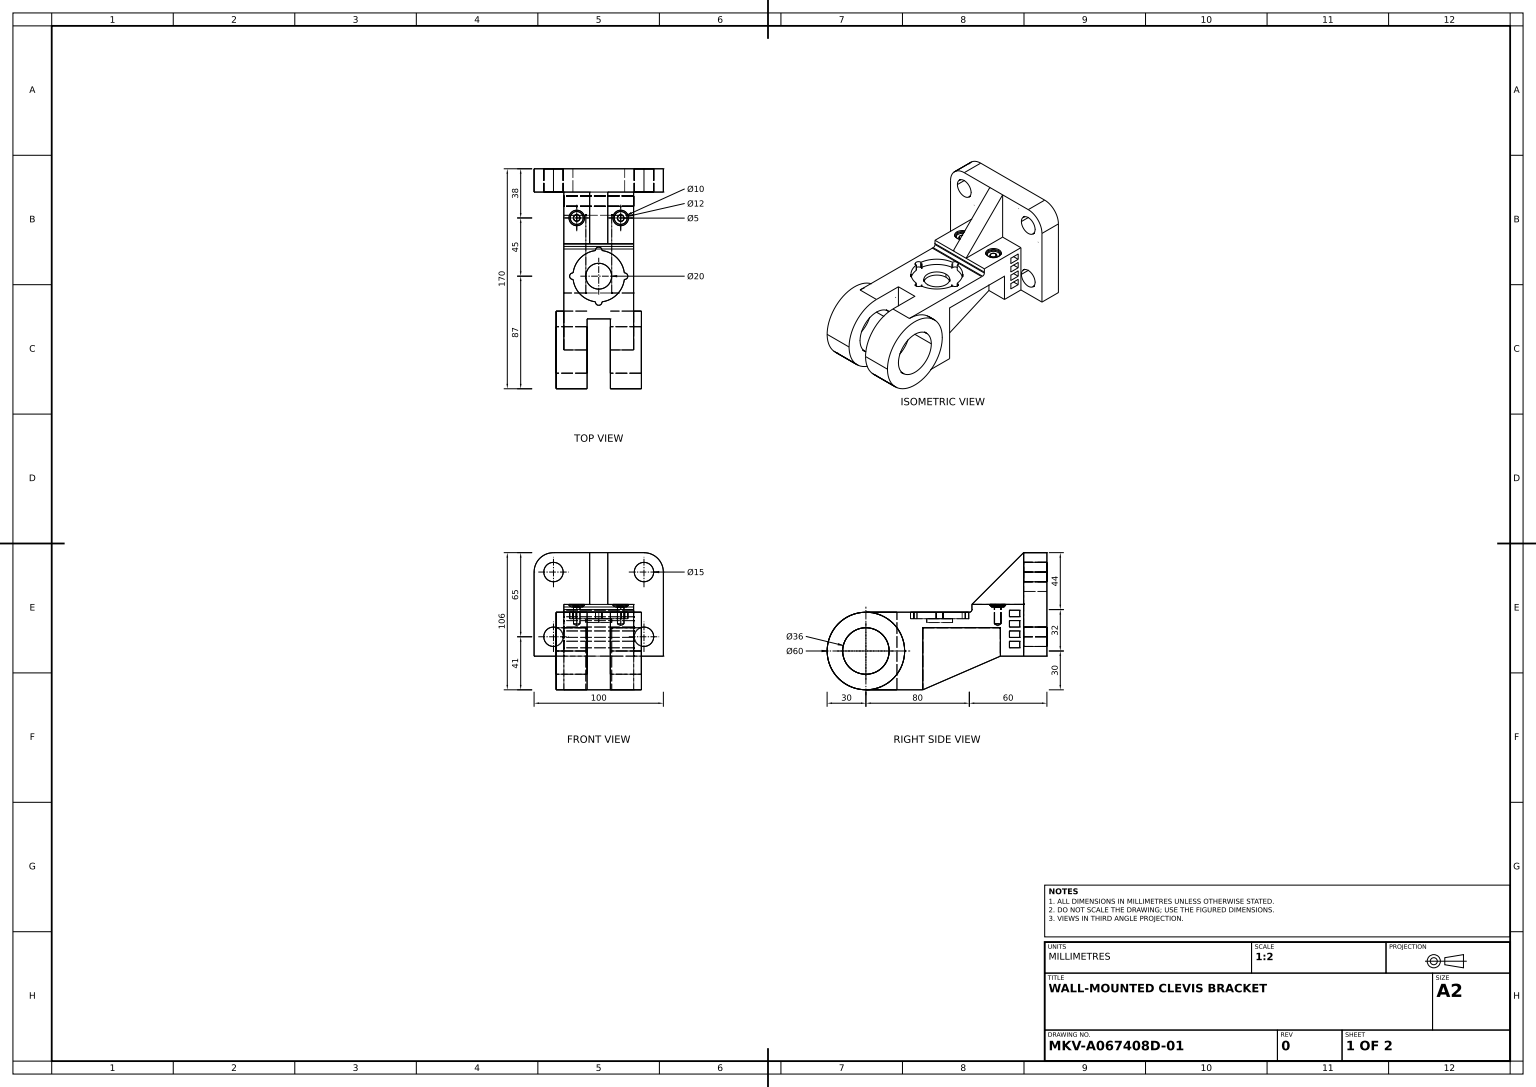
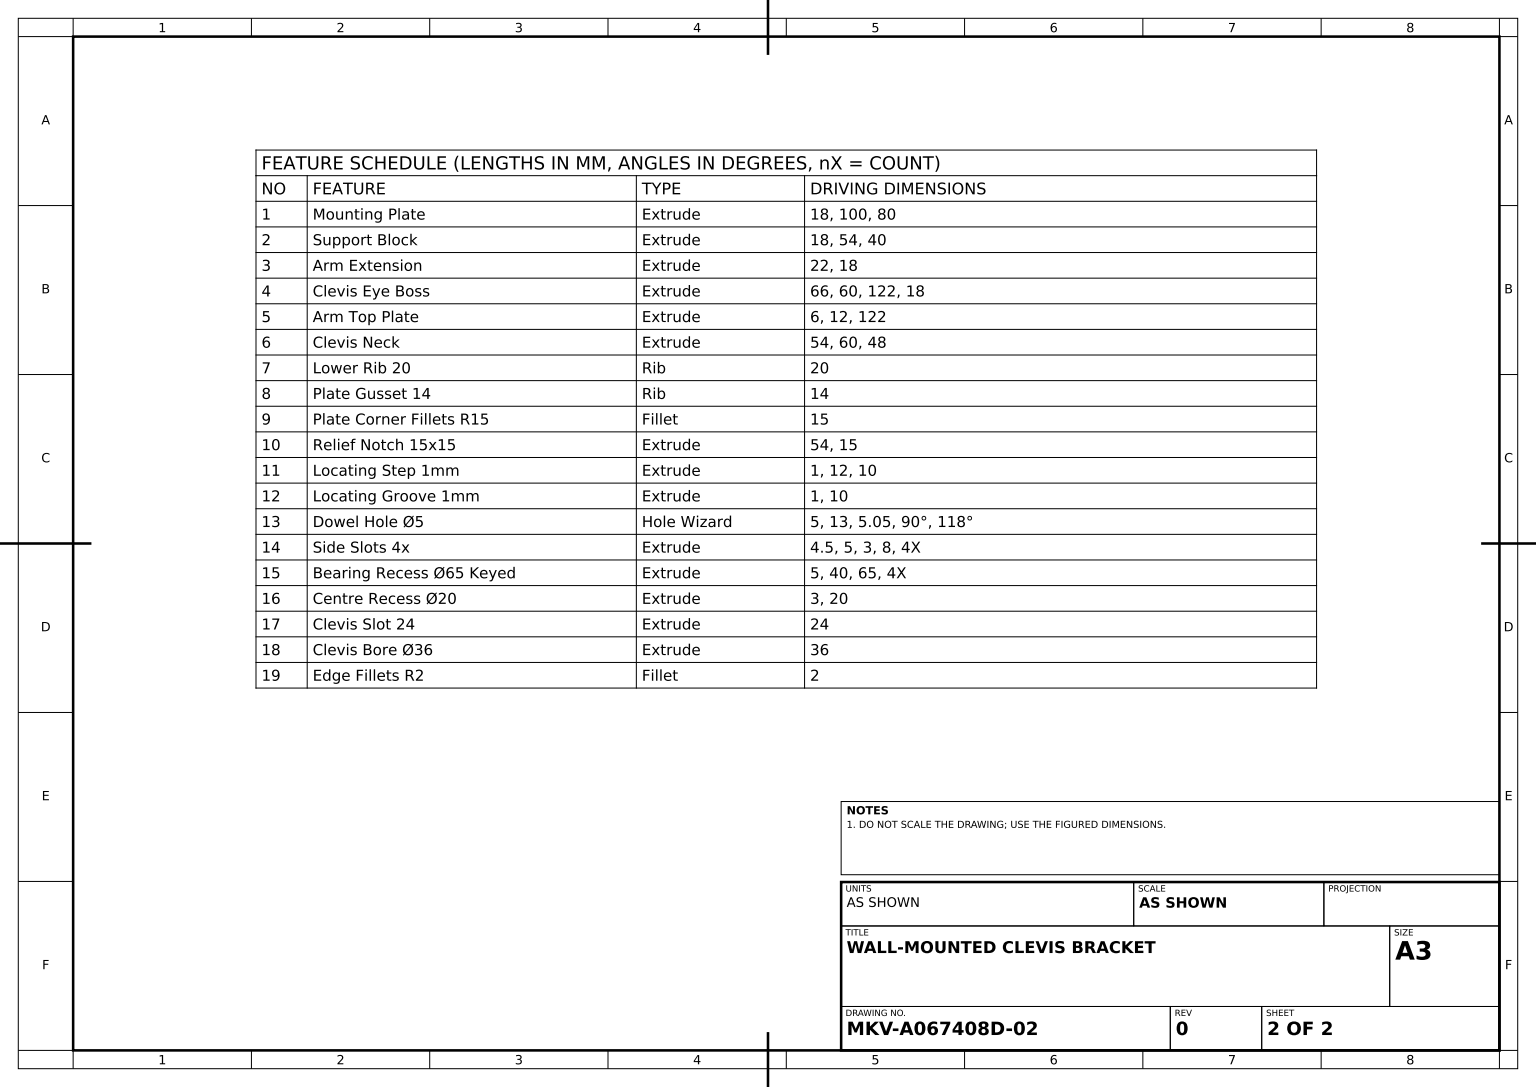
solid
v1 (-35,40,18)
v2 (-50,25,18)
e1 v1 v2 CIRCLE(AX(P(-35,25,18),D(0,0,1),D(-1,0,0)),15)
v3 (-35,40,0)
e2 v3 v1 LINE
v4 (-50,25,0)
e3 v4 v3 CIRCLE(AX(P(-35,25,0),D(0,0,-1),D(-1,0,0)),15)
e4 v2 v4 LINE
face CYL(AX(P(-35,25,18),D(0,0,-1),D(-1,0,0)),15) [-e1 -e2 -e3 -e4]
v5 (27,-12.5,29)
v6 (-27,-12.5,29)
e5 v5 v6 LINE
v7 (-27,-12.5,21)
e6 v6 v7 LINE
v8 (27,-12.5,21)
e7 v8 v7 LINE
e8 v5 v8 LINE
face PLANE(AX(P(50,-12.5,21),D(0,1,0),D(0,0,1))) rev [e5 e6 -e7 -e8]
v9 (20,-11,85.5)
v10 (20,-11,80.5)
e9 v9 v10 CIRCLE(AX(P(20,-11,83),D(0,1,0),D(0,0,1)),2.5)
v11 (20,-6,85.5)
e10 v9 v11 LINE
v12 (20,-6,80.5)
e11 v11 v12 CIRCLE(AX(P(20,-6,83),D(0,1,0),D(0,0,1)),2.5)
e12 v10 v12 LINE
face CYL(AX(P(20,-11,83),D(0,1,0),D(0,0,1)),2.5) rev [-e9 e10 e11 -e12]
v13 (27,-25.5,21)
v14 (27,-25.5,29)
e13 v13 v14 LINE
v15 (-27,-25.5,21)
e14 v13 v15 LINE
v16 (-27,-25.5,29)
e15 v15 v16 LINE
e16 v14 v16 LINE
face PLANE(AX(P(50,-25.5,21),D(0,-1,0),D(0,0,-1))) rev [-e13 e14 e15 -e16]
v17 (33,-36,122)
v18 (9,-36,122)
e17 v17 v18 LINE
v19 (9,-36,158)
e18 v19 v18 CIRCLE(AX(P(9,-36,140),D(1,0,0),D(0,0,-1)),18)
v20 (33,-36,158)
e19 v20 v19 LINE
e20 v20 v17 CIRCLE(AX(P(33,-36,140),D(1,0,0),D(0,0,-1)),18)
face CYL(AX(P(50,-36,140),D(-1,0,0),D(0,0,1)),18) rev [e17 -e18 -e19 e20]
v21 (27,-20.5,29)
v22 (-27,-20.5,29)
e21 v21 v22 LINE
e22 v14 v21 LINE
e23 v16 v22 LINE
face PLANE(AX(P(50,-20.5,29),D(0,0,1),D(1,0,0))) rev [-e21 -e22 e16 e23]
v23 (-17,-2,35.475)
v24 (-17,-2,40.525)
e24 v23 v24 CIRCLE(AX(P(-17,-2,38),D(0,1,0),D(0,0,1)),2.525)
v25 (-17,-2.025,40.5)
e25 v25 v24 LINE
v26 (-17,-2.025,35.5)
e26 v26 v25 CIRCLE(AX(P(-17,-2.025,38),D(0,1,0),D(0,0,1)),2.5)
e27 v26 v23 LINE
face CONE(AX(P(-17,-2,38),D(0,1,0),D(0,0,1)),2.525,0.785398163) rev [e24 -e25 -e26 e27]
v27 (12,-2,38)
v28 (12,-1,38)
e28 v27 v28 LINE
v29 (22,-2,38)
e29 v29 v27 CIRCLE(AX(P(17,-2,38),D(0,1,0),D(-1,0,0)),5)
v30 (22,-1,38)
e30 v29 v30 LINE
e31 v30 v28 CIRCLE(AX(P(17,-1,38),D(0,1,0),D(-1,0,0)),5)
face CYL(AX(P(17,-2,38),D(0,1,0),D(-1,0,0)),5) rev [-e28 -e29 e30 e31]
v31 (19.84375,-6,80.504888)
e32 v12 v31 CIRCLE(AX(P(20,-6,83),D(0,1,0),D(0,0,1)),2.5)
v32 (19.84375,-11,80.504888)
e33 v32 v31 LINE
e34 v10 v32 CIRCLE(AX(P(20,-11,83),D(0,1,0),D(0,0,1)),2.5)
face CYL(AX(P(20,-11,83),D(0,1,0),D(0,0,1)),2.5) rev [e32 -e33 -e34 e12]
v33 (17,-16.502152,38.121872)
v34 (17,-15,40.621872)
e35 v33 v34 LINE
v35 (17,-15,35.621872)
e36 v33 v35 LINE
e37 v35 v34 CIRCLE(AX(P(17,-15,38.121872),D(0,1,0),D(0,0,1)),2.5)
face CONE(AX(P(17,-15,38.121872),D(0,1,0),D(0,0,1)),2.5,1.029744259) rev [-e35 e36 e37]
v36 (-33,-36,110)
v37 (-33,-36,170)
e38 v36 v37 CIRCLE(AX(P(-33,-36,140),D(1,0,0),D(0,0,-1)),30)
e39 v37 v36 CIRCLE(AX(P(-33,-36,140),D(1,0,0),D(0,0,-1)),30)
v38 (-33,-36,122)
v39 (-33,-36,158)
e40 v38 v39 CIRCLE(AX(P(-33,-36,140),D(-1,0,0),D(0,0,1)),18)
e41 v39 v38 CIRCLE(AX(P(-33,-36,140),D(-1,0,0),D(0,0,1)),18)
face PLANE(AX(P(-33,-36,140),D(1,0,0),D(0,0,-1))) rev [-e38 -e39] [-e40 -e41]
v40 (-42.5,-25,18)
v41 (-27.5,-25,18)
e42 v40 v41 CIRCLE(AX(P(-35,-25,18),D(0,0,1),D(1,0,0)),7.5)
e43 v41 v40 CIRCLE(AX(P(-35,-25,18),D(0,0,1),D(1,0,0)),7.5)
v42 (-27,0,18)
v43 (-27,-40,18)
e44 v42 v43 LINE
v44 (-7,0,18)
e45 v44 v42 LINE
v45 (-7,40,18)
e46 v45 v44 LINE
e47 v45 v1 LINE
v46 (-50,-40,18)
e48 v2 v46 LINE
e49 v46 v43 LINE
v47 (-42.5,25,18)
v48 (-27.5,25,18)
e50 v47 v48 CIRCLE(AX(P(-35,25,18),D(0,0,1),D(1,0,0)),7.5)
e51 v48 v47 CIRCLE(AX(P(-35,25,18),D(0,0,1),D(1,0,0)),7.5)
face PLANE(AX(P(0,0,18),D(0,0,-1),D(-1,0,0))) rev [-e42 -e43] [-e44 -e45 -e46 e47 e1 e48 e49] [-e50 -e51]
v49 (10,-40,36)
v50 (10,-66,96)
e52 v49 v50 LINE
v51 (-10,-66,96)
e53 v50 v51 LINE
v52 (-10,-40,36)
e54 v52 v51 LINE
e55 v49 v52 LINE
face PLANE(AX(P(0,-40,36),D(0,0.917555625,0.397607438),D(0,-0.397607438,0.917555625))) rev [e52 e53 -e54 -e55]
v53 (-27,-40,36)
e56 v53 v52 LINE
v54 (-10,-18,36)
e57 v54 v52 LINE
v55 (-27,-18,36)
e58 v55 v54 LINE
e59 v55 v53 LINE
face PLANE(AX(P(0,0,36),D(0,0,-1),D(-1,0,0))) rev [e56 -e57 -e58 e59]
v56 (-9,-36,170)
e60 v56 v37 LINE
v57 (-27,-36,110)
e61 v57 v36 LINE
v58 (-27,-66,140)
e62 v57 v58 CIRCLE(AX(P(-27,-36,140),D(-1,0,0),D(0,0,-1)),30)
v59 (-9,-66,140)
e63 v59 v58 LINE
e64 v59 v56 CIRCLE(AX(P(-9,-36,140),D(-1,0,0),D(0,0,1)),30)
face CYL(AX(P(33,-36,140),D(-1,0,0),D(0,0,1)),30) [e60 e39 -e61 e62 -e63 e64]
v60 (11,-1,38)
v61 (11,0,38)
e65 v60 v61 LINE
v62 (23,-1,38)
e66 v62 v60 CIRCLE(AX(P(17,-1,38),D(0,1,0),D(-1,0,0)),6)
v63 (23,0,38)
e67 v62 v63 LINE
e68 v63 v61 CIRCLE(AX(P(17,0,38),D(0,1,0),D(-1,0,0)),6)
face CYL(AX(P(17,-1,38),D(0,1,0),D(-1,0,0)),6) rev [-e65 -e66 e67 e68]
v64 (-27,-9.5,21)
v65 (-27,-9.5,29)
e69 v64 v65 LINE
v66 (27,-9.5,29)
e70 v66 v65 LINE
v67 (27,-9.5,21)
e71 v67 v66 LINE
e72 v67 v64 LINE
face PLANE(AX(P(50,-9.5,21),D(0,-1,0),D(0,0,-1))) rev [e69 -e70 -e71 e72]
v68 (10,-18,36)
v69 (27,-18,36)
e73 v68 v69 LINE
e74 v68 v49 LINE
v70 (27,-40,36)
e75 v49 v70 LINE
e76 v70 v69 LINE
face PLANE(AX(P(0,0,36),D(0,0,-1),D(-1,0,0))) rev [-e73 e74 e75 e76]
v71 (42.5,-25,18)
v72 (27.5,-25,18)
e77 v71 v72 CIRCLE(AX(P(35,-25,18),D(0,0,1),D(1,0,0)),7.5)
e78 v72 v71 CIRCLE(AX(P(35,-25,18),D(0,0,1),D(1,0,0)),7.5)
v73 (27.5,25,18)
v74 (42.5,25,18)
e79 v73 v74 CIRCLE(AX(P(35,25,18),D(0,0,1),D(1,0,0)),7.5)
e80 v74 v73 CIRCLE(AX(P(35,25,18),D(0,0,1),D(1,0,0)),7.5)
v75 (27,0,18)
v76 (7,0,18)
e81 v75 v76 LINE
v77 (27,-40,18)
e82 v77 v75 LINE
v78 (50,-40,18)
e83 v77 v78 LINE
v79 (50,25,18)
e84 v78 v79 LINE
v80 (35,40,18)
e85 v79 v80 CIRCLE(AX(P(35,25,18),D(0,0,1),D(-1,0,0)),15)
v81 (7,40,18)
e86 v80 v81 LINE
e87 v81 v76 LINE
face PLANE(AX(P(0,0,18),D(0,0,-1),D(-1,0,0))) rev [-e77 -e78] [-e79 -e80] [-e81 -e82 e83 e84 e85 e86 e87]
v82 (-17,-15,35.5)
v83 (-17,-15,40.5)
e88 v82 v83 CIRCLE(AX(P(-17,-15,38),D(0,1,0),D(0,0,1)),2.5)
e89 v82 v26 LINE
e90 v83 v25 LINE
face CYL(AX(P(-17,-2,38),D(0,1,0),D(0,0,1)),2.5) rev [-e88 e89 e26 -e90]
v84 (-9,-36,122)
e91 v84 v38 LINE
v85 (-9,-36,158)
e92 v85 v39 LINE
e93 v84 v85 CIRCLE(AX(P(-9,-36,140),D(-1,0,0),D(0,0,1)),18)
face CYL(AX(P(50,-36,140),D(-1,0,0),D(0,0,1)),18) rev [e91 e40 -e92 -e93]
v86 (27,-66,140)
v87 (27,-36,110)
e94 v86 v87 CIRCLE(AX(P(27,-36,140),D(1,0,0),D(0,-1,0)),30)
v88 (33,-36,110)
e95 v88 v87 LINE
v89 (33,-36,170)
e96 v89 v88 CIRCLE(AX(P(33,-36,140),D(1,0,0),D(0,0,-1)),30)
v90 (9,-36,170)
e97 v89 v90 LINE
v91 (9,-66,140)
e98 v90 v91 CIRCLE(AX(P(9,-36,140),D(1,0,0),D(0,0,-1)),30)
e99 v86 v91 LINE
face CYL(AX(P(33,-36,140),D(-1,0,0),D(0,0,1)),30) [e94 -e95 -e96 e97 e98 -e99]
v92 (27,-28.5,21)
v93 (27,-33.5,21)
e100 v92 v93 LINE
v94 (-27,-28.5,21)
e101 v92 v94 LINE
v95 (-27,-33.5,21)
e102 v94 v95 LINE
e103 v93 v95 LINE
face PLANE(AX(P(50,-28.5,21),D(0,0,-1),D(-1,0,0))) rev [-e100 e101 e102 -e103]
v96 (-7,0,58)
e104 v44 v96 LINE
v97 (-27,0,58)
e105 v97 v42 LINE
e106 v96 v97 LINE
v98 (-11,0,38)
v99 (-23,0,38)
e107 v98 v99 CIRCLE(AX(P(-17,0,38),D(0,1,0),D(-1,0,0)),6)
e108 v99 v98 CIRCLE(AX(P(-17,0,38),D(0,1,0),D(-1,0,0)),6)
face PLANE(AX(P(-27,0,36),D(0,-1,0),D(1,0,0))) rev [-e104 e45 -e105 -e106] [-e107 -e108]
v100 (-20,-6,80.5)
v101 (-20,-6,85.5)
e109 v100 v101 CIRCLE(AX(P(-20,-6,83),D(0,1,0),D(0,0,1)),2.5)
v102 (-20,-11,85.5)
e110 v102 v101 LINE
v103 (-20,-11,80.5)
e111 v103 v102 CIRCLE(AX(P(-20,-11,83),D(0,1,0),D(0,0,1)),2.5)
e112 v103 v100 LINE
face CYL(AX(P(-20,-11,83),D(0,1,0),D(0,0,1)),2.5) rev [e109 -e110 -e111 e112]
v104 (17,-2,40.646872)
v105 (17,-2,35.596872)
e113 v104 v105 CIRCLE(AX(P(17,-2,38.121872),D(0,1,0),D(0,0,1)),2.525)
v106 (17,-2.025,35.621872)
e114 v106 v105 LINE
v107 (17,-2.025,40.621872)
e115 v107 v106 CIRCLE(AX(P(17,-2.025,38.121872),D(0,1,0),D(0,0,1)),2.5)
e116 v107 v104 LINE
face CONE(AX(P(17,-2,38.121872),D(0,1,0),D(0,0,1)),2.525,0.785398163) rev [e113 -e114 -e115 e116]
v108 (50,-40,0)
e117 v78 v108 LINE
v109 (50,25,0)
e118 v108 v109 LINE
e119 v109 v79 LINE
face PLANE(AX(P(50,-40,18),D(-1,0,0),D(0,0,1))) rev [e117 e118 e119 -e84]
e120 v45 v96 LINE
face PLANE(AX(P(-7,-13,85),D(1,0,0),D(0,0,-1))) rev [e46 e104 -e120]
v110 (-27,-6,60)
v111 (-27,-4,58)
e121 v110 v111 CIRCLE(AX(P(-27,-4,60),D(1,0,0),D(0,0,-1)),2)
v112 (27,-6,60)
e122 v112 v110 LINE
v113 (27,-4,58)
e123 v113 v112 CIRCLE(AX(P(27,-4,60),D(-1,0,0),D(0,-1,0)),2)
e124 v111 v113 LINE
face CYL(AX(P(0,-4,60),D(1,0,0),D(0,0,-1)),2) rev [-e121 -e122 -e123 -e124]
e125 v61 v63 CIRCLE(AX(P(17,0,38),D(0,1,0),D(-1,0,0)),6)
e126 v60 v62 CIRCLE(AX(P(17,-1,38),D(0,1,0),D(-1,0,0)),6)
face CYL(AX(P(17,-1,38),D(0,1,0),D(-1,0,0)),6) rev [e65 e125 -e67 -e126]
v114 (2.495112,-11,102.84375)
v115 (19.84375,-11,85.495112)
e127 v114 v115 CIRCLE(AX(P(0,-11,83),D(0,1,0),D(0,0,1)),20)
v116 (2.495112,-6,102.84375)
e128 v114 v116 LINE
v117 (19.84375,-6,85.495112)
e129 v116 v117 CIRCLE(AX(P(0,-6,83),D(0,1,0),D(0,0,1)),20)
e130 v115 v117 LINE
face CYL(AX(P(0,-11,83),D(0,1,0),D(0,0,1)),20) rev [-e127 e128 e129 -e130]
e131 v83 v82 CIRCLE(AX(P(-17,-15,38),D(0,1,0),D(0,0,1)),2.5)
e132 v25 v26 CIRCLE(AX(P(-17,-2.025,38),D(0,1,0),D(0,0,1)),2.5)
face CYL(AX(P(-17,-2,38),D(0,1,0),D(0,0,1)),2.5) rev [-e131 e90 e132 -e89]
v118 (27.5,25,0)
v119 (42.5,25,0)
e133 v118 v119 CIRCLE(AX(P(35,25,0),D(0,0,-1),D(-1,0,0)),7.5)
e134 v119 v74 LINE
e135 v118 v73 LINE
face CYL(AX(P(35,25,-36),D(0,0,1),D(1,0,0)),7.5) rev [e133 e134 e80 -e135]
e136 v28 v30 CIRCLE(AX(P(17,-1,38),D(0,1,0),D(-1,0,0)),5)
e137 v27 v29 CIRCLE(AX(P(17,-2,38),D(0,1,0),D(-1,0,0)),5)
face CYL(AX(P(17,-2,38),D(0,1,0),D(-1,0,0)),5) rev [e136 -e30 -e137 e28]
v120 (27,-66,96)
e138 v120 v50 LINE
v121 (10,-18,96)
e139 v121 v50 LINE
v122 (27,-18,96)
e140 v122 v121 LINE
e141 v122 v120 LINE
face PLANE(AX(P(27,-18,96),D(0,0,-1),D(-1,0,0))) [e138 -e139 -e140 e141]
v123 (-27,-17.5,21)
e142 v7 v123 LINE
v124 (27,-17.5,21)
e143 v124 v123 LINE
e144 v8 v124 LINE
face PLANE(AX(P(50,-12.5,21),D(0,0,-1),D(-1,0,0))) rev [e7 e142 -e143 -e144]
v125 (-11,-1,38)
e145 v125 v98 LINE
v126 (-23,-1,38)
e146 v126 v125 CIRCLE(AX(P(-17,-1,38),D(0,1,0),D(-1,0,0)),6)
e147 v126 v99 LINE
face CYL(AX(P(-17,-1,38),D(0,1,0),D(-1,0,0)),6) rev [e108 -e145 -e146 e147]
v127 (-10,-18,96)
e148 v127 v51 LINE
e149 v127 v54 LINE
face PLANE(AX(P(-10,-13,85),D(1,0,0),D(0,0,-1))) rev [-e148 e149 e57 e54]
v128 (-17,-16.502152,38)
e150 v128 v82 LINE
e151 v128 v83 LINE
face CONE(AX(P(-17,-15,38),D(0,1,0),D(0,0,1)),2.5,1.029744259) rev [e131 -e150 e151]
e152 v117 v11 CIRCLE(AX(P(20,-6,83),D(0,1,0),D(0,0,1)),2.5)
e153 v115 v9 CIRCLE(AX(P(20,-11,83),D(0,1,0),D(0,0,1)),2.5)
face CYL(AX(P(20,-11,83),D(0,1,0),D(0,0,1)),2.5) rev [e152 -e10 -e153 e130]
e154 v34 v35 CIRCLE(AX(P(17,-15,38.121872),D(0,1,0),D(0,0,1)),2.5)
face CONE(AX(P(17,-15,38.121872),D(0,1,0),D(0,0,1)),2.5,1.029744259) rev [-e36 e35 e154]
v129 (27,-28.5,29)
v130 (-27,-28.5,29)
e155 v129 v130 LINE
v131 (27,-33.5,29)
e156 v131 v129 LINE
v132 (-27,-33.5,29)
e157 v131 v132 LINE
e158 v132 v130 LINE
face PLANE(AX(P(50,-28.5,29),D(0,0,1),D(1,0,0))) rev [-e155 -e156 e157 e158]
e159 v125 v126 CIRCLE(AX(P(-17,-1,38),D(0,1,0),D(-1,0,0)),6)
face CYL(AX(P(-17,-1,38),D(0,1,0),D(-1,0,0)),6) rev [e145 e107 -e147 -e159]
e160 v119 v118 CIRCLE(AX(P(35,25,0),D(0,0,-1),D(-1,0,0)),7.5)
face CYL(AX(P(35,25,-36),D(0,0,1),D(1,0,0)),7.5) rev [-e134 e160 e135 e79]
e161 v85 v84 CIRCLE(AX(P(-9,-36,140),D(-1,0,0),D(0,0,1)),18)
v133 (-9,-66,116)
v134 (-9,-6,116)
e162 v133 v134 LINE
v135 (-9,-6,140)
e163 v134 v135 LINE
e164 v56 v135 CIRCLE(AX(P(-9,-36,140),D(-1,0,0),D(0,0,1)),30)
e165 v133 v59 LINE
face PLANE(AX(P(-9,-66,116),D(-1,0,0),D(0,0,1))) rev [e161 e93] [e162 e163 -e164 -e64 -e165]
v136 (27,-17.5,29)
e166 v124 v136 LINE
v137 (-27,-17.5,29)
e167 v123 v137 LINE
e168 v136 v137 LINE
face PLANE(AX(P(50,-17.5,21),D(0,-1,0),D(0,0,-1))) rev [-e166 e143 e167 -e168]
v138 (35,40,0)
e169 v80 v138 LINE
e170 v138 v109 CIRCLE(AX(P(35,25,0),D(0,0,-1),D(-1,0,0)),15)
face CYL(AX(P(35,25,18),D(0,0,-1),D(-1,0,0)),15) [-e169 -e85 -e119 -e170]
v139 (42.5,-25,0)
v140 (27.5,-25,0)
e171 v139 v140 CIRCLE(AX(P(35,-25,0),D(0,0,-1),D(-1,0,0)),7.5)
e172 v140 v139 CIRCLE(AX(P(35,-25,0),D(0,0,-1),D(-1,0,0)),7.5)
v141 (-50,-40,0)
e173 v141 v108 LINE
e174 v4 v141 LINE
e175 v138 v3 LINE
v142 (-27.5,25,0)
v143 (-42.5,25,0)
e176 v142 v143 CIRCLE(AX(P(-35,25,0),D(0,0,-1),D(-1,0,0)),7.5)
e177 v143 v142 CIRCLE(AX(P(-35,25,0),D(0,0,-1),D(-1,0,0)),7.5)
v144 (-42.5,-25,0)
v145 (-27.5,-25,0)
e178 v144 v145 CIRCLE(AX(P(-35,-25,0),D(0,0,-1),D(-1,0,0)),7.5)
e179 v145 v144 CIRCLE(AX(P(-35,-25,0),D(0,0,-1),D(-1,0,0)),7.5)
face PLANE(AX(P(0,0,0),D(0,0,-1),D(-1,0,0))) [-e160 -e133] [-e171 -e172] [e170 -e118 -e173 -e174 e3 -e175] [-e176 -e177] [-e178 -e179]
e180 v81 v45 LINE
face PLANE(AX(P(-50,40,18),D(0,-1,0),D(0,0,-1))) rev [e2 -e47 -e180 -e86 e169 e175]
face CYL(AX(P(50,-36,140),D(-1,0,0),D(0,0,1)),18) rev [e92 e41 -e91 -e161]
v146 (9,-66,116)
e181 v146 v91 LINE
e182 v146 v133 LINE
v147 (-27,-66,96)
e183 v147 v58 LINE
e184 v51 v147 LINE
e185 v120 v86 LINE
face PLANE(AX(P(27,-66,96),D(0,-1,0),D(0,0,-1))) [-e181 e182 e165 e63 -e183 -e184 -e53 -e138 e185 e99]
e186 v53 v43 LINE
e187 v46 v141 LINE
e188 v70 v77 LINE
face PLANE(AX(P(-50,-40,18),D(0,1,0),D(0,0,1))) rev [e186 -e49 e187 e173 -e117 -e83 -e188 -e75 e55 -e56]
v148 (-27,-4.5,29)
e189 v65 v148 LINE
v149 (27,-4.5,29)
e190 v149 v148 LINE
e191 v66 v149 LINE
face PLANE(AX(P(50,-4.5,29),D(0,0,1),D(1,0,0))) rev [e189 -e190 -e191 e70]
e192 v143 v47 LINE
e193 v142 v48 LINE
face CYL(AX(P(-35,25,-36),D(0,0,1),D(1,0,0)),7.5) rev [e176 e192 e50 -e193]
e194 v17 v20 CIRCLE(AX(P(33,-36,140),D(1,0,0),D(0,0,-1)),18)
e195 v18 v19 CIRCLE(AX(P(9,-36,140),D(1,0,0),D(0,0,-1)),18)
face CYL(AX(P(50,-36,140),D(-1,0,0),D(0,0,1)),18) rev [-e17 e194 e19 -e195]
e196 v144 v40 LINE
e197 v145 v41 LINE
face CYL(AX(P(-35,-25,-36),D(0,0,1),D(1,0,0)),7.5) rev [-e196 e178 e197 e43]
face PLANE(AX(P(17,-1,38),D(0,1,0),D(-1,0,0))) [e66 e126] [-e31 -e136]
v150 (9,-6,140)
e198 v150 v90 CIRCLE(AX(P(9,-36,140),D(1,0,0),D(0,0,-1)),30)
v151 (9,-6,116)
e199 v150 v151 LINE
e200 v146 v151 LINE
face PLANE(AX(P(9,-66,116),D(1,0,0),D(0,0,-1))) rev [-e98 -e198 e199 -e200 e181] [e195 e18]
v152 (-2.495112,-11,63.15625)
v153 (-2.495112,-6,63.15625)
e201 v152 v153 LINE
v154 (-19.84375,-6,80.504888)
e202 v153 v154 CIRCLE(AX(P(0,-6,83),D(0,1,0),D(0,0,1)),20)
v155 (-19.84375,-11,80.504888)
e203 v155 v154 LINE
e204 v152 v155 CIRCLE(AX(P(0,-11,83),D(0,1,0),D(0,0,1)),20)
face CYL(AX(P(0,-11,83),D(0,1,0),D(0,0,1)),20) rev [e201 e202 -e203 -e204]
e205 v140 v72 LINE
e206 v139 v71 LINE
face CYL(AX(P(35,-25,-36),D(0,0,1),D(1,0,0)),7.5) rev [-e205 e172 e206 e77]
v156 (2.495112,-11,63.15625)
e207 v32 v156 CIRCLE(AX(P(0,-11,83),D(0,1,0),D(0,0,1)),20)
v157 (2.495112,-6,63.15625)
e208 v31 v157 CIRCLE(AX(P(0,-6,83),D(0,1,0),D(0,0,1)),20)
e209 v156 v157 LINE
face CYL(AX(P(0,-11,83),D(0,1,0),D(0,0,1)),20) rev [-e207 e33 e208 -e209]
e210 v95 v132 LINE
e211 v93 v131 LINE
face PLANE(AX(P(50,-33.5,21),D(0,-1,0),D(0,0,-1))) rev [e210 -e157 -e211 e103]
e212 v129 v92 LINE
e213 v130 v94 LINE
face PLANE(AX(P(50,-28.5,21),D(0,1,0),D(0,0,1))) rev [-e101 -e212 e155 e213]
v158 (0,-11,105.5)
e214 v158 v114 CIRCLE(AX(P(0,-11,103),D(0,1,0),D(0,0,1)),2.5)
v159 (0,-6,105.5)
e215 v158 v159 LINE
e216 v159 v116 CIRCLE(AX(P(0,-6,103),D(0,1,0),D(0,0,1)),2.5)
face CYL(AX(P(0,-11,103),D(0,1,0),D(0,0,1)),2.5) rev [-e128 -e214 e215 e216]
e217 v121 v68 LINE
face PLANE(AX(P(10,-13,85),D(1,0,0),D(0,0,-1))) [-e52 -e74 -e217 e139]
e218 v122 v69 LINE
face PLANE(AX(P(-27,-18,58),D(0,1,0),D(0,0,1))) rev [-e218 e140 e217 e73]
v160 (-27,-6,140)
e219 v160 v135 LINE
e220 v160 v57 CIRCLE(AX(P(-27,-36,140),D(-1,0,0),D(0,0,-1)),30)
face CYL(AX(P(33,-36,140),D(-1,0,0),D(0,0,1)),30) [e164 -e219 e220 e61 e38 -e60]
v161 (0,-14,93)
v162 (0,-14,73)
e221 v161 v162 CIRCLE(AX(P(0,-14,83),D(0,1,0),D(0,0,1)),10)
e222 v162 v161 CIRCLE(AX(P(0,-14,83),D(0,1,0),D(0,0,1)),10)
face PLANE(AX(P(0,-14,83),D(0,1,0),D(0,0,1))) [e221 e222]
e223 v106 v107 CIRCLE(AX(P(17,-2.025,38.121872),D(0,1,0),D(0,0,1)),2.5)
e224 v34 v107 LINE
e225 v35 v106 LINE
face CYL(AX(P(17,-2,38.121872),D(0,1,0),D(0,0,1)),2.5) rev [e223 -e224 -e37 e225]
v163 (27,-20.5,21)
e226 v163 v13 LINE
v164 (-27,-20.5,21)
e227 v163 v164 LINE
e228 v164 v15 LINE
face PLANE(AX(P(50,-20.5,21),D(0,0,-1),D(-1,0,0))) rev [-e226 e227 e228 -e14]
v165 (-27,-18,96)
e229 v165 v55 LINE
e230 v165 v147 LINE
e231 v110 v160 LINE
e232 v97 v111 LINE
v166 (-27,-4.5,21)
e233 v166 v64 LINE
e234 v148 v166 LINE
e235 v22 v164 LINE
e236 v137 v6 LINE
face PLANE(AX(P(-27,-40,36),D(1,0,0),D(0,0,-1))) rev [-e213 -e158 -e210 -e102] [-e186 -e59 -e229 e230 e183 -e62 -e220 -e231 e121 -e232 e105 e44] [-e189 -e69 -e233 -e234] [-e235 -e23 -e15 -e228] [-e142 -e6 -e236 -e167]
e237 v136 v5 LINE
face PLANE(AX(P(50,-12.5,29),D(0,0,1),D(1,0,0))) rev [-e5 -e237 e168 e236]
e238 v151 v134 LINE
face PLANE(AX(P(-9,-66,116),D(0,0,-1),D(-1,0,0))) rev [-e182 e200 e238 -e162]
v167 (7,0,58)
e239 v167 v96 LINE
e240 v81 v167 LINE
face PLANE(AX(P(0,40,18),D(0,0.707106781,0.707106781),D(0,-0.707106781,0.707106781))) [-e239 -e240 e180 e120]
e241 v24 v23 CIRCLE(AX(P(-17,-2,38),D(0,1,0),D(0,0,1)),2.525)
v168 (-12,-2,38)
v169 (-22,-2,38)
e242 v168 v169 CIRCLE(AX(P(-17,-2,38),D(0,1,0),D(-1,0,0)),5)
e243 v169 v168 CIRCLE(AX(P(-17,-2,38),D(0,1,0),D(-1,0,0)),5)
face PLANE(AX(P(-17,-2,38),D(0,1,0),D(-1,0,0))) [-e24 -e241] [e242 e243]
v170 (27,-4.5,21)
e244 v170 v67 LINE
e245 v170 v166 LINE
face PLANE(AX(P(50,-4.5,21),D(0,0,-1),D(-1,0,0))) rev [e233 -e72 -e244 e245]
e246 v76 v167 LINE
face PLANE(AX(P(7,-13,85),D(1,0,0),D(0,0,-1))) [-e246 -e87 e240]
v171 (-19.84375,-6,85.495112)
e247 v101 v171 CIRCLE(AX(P(-20,-6,83),D(0,1,0),D(0,0,1)),2.5)
v172 (-19.84375,-11,85.495112)
e248 v172 v171 LINE
e249 v102 v172 CIRCLE(AX(P(-20,-11,83),D(0,1,0),D(0,0,1)),2.5)
face CYL(AX(P(-20,-11,83),D(0,1,0),D(0,0,1)),2.5) rev [e110 e247 -e248 -e249]
e250 v88 v89 CIRCLE(AX(P(33,-36,140),D(1,0,0),D(0,0,-1)),30)
face PLANE(AX(P(33,-36,140),D(1,0,0),D(0,0,-1))) [-e194 -e20] [e250 e96]
e251 v149 v170 LINE
face PLANE(AX(P(50,-4.5,21),D(0,1,0),D(0,0,1))) rev [e234 -e245 -e251 e190]
v173 (0,-11,73)
e252 v162 v173 LINE
v174 (0,-11,93)
e253 v173 v174 CIRCLE(AX(P(0,-11,83),D(0,1,0),D(0,0,1)),10)
e254 v161 v174 LINE
face CYL(AX(P(0,-14,83),D(0,1,0),D(0,0,1)),10) rev [-e222 e252 e253 -e254]
e255 v105 v104 CIRCLE(AX(P(17,-2,38.121872),D(0,1,0),D(0,0,1)),2.525)
face CONE(AX(P(17,-2,38.121872),D(0,1,0),D(0,0,1)),2.525,0.785398163) rev [e255 -e116 -e223 e114]
face CYL(AX(P(-35,25,-36),D(0,0,1),D(1,0,0)),7.5) rev [e193 e51 -e192 e177]
v175 (-12,-1,38)
e256 v168 v175 LINE
v176 (-22,-1,38)
e257 v175 v176 CIRCLE(AX(P(-17,-1,38),D(0,1,0),D(-1,0,0)),5)
e258 v169 v176 LINE
face CYL(AX(P(-17,-2,38),D(0,1,0),D(-1,0,0)),5) rev [e256 e257 -e258 -e242]
v177 (-2.495112,-6,102.84375)
e259 v171 v177 CIRCLE(AX(P(0,-6,83),D(0,1,0),D(0,0,1)),20)
v178 (-2.495112,-11,102.84375)
e260 v178 v177 LINE
e261 v172 v178 CIRCLE(AX(P(0,-11,83),D(0,1,0),D(0,0,1)),20)
face CYL(AX(P(0,-11,83),D(0,1,0),D(0,0,1)),20) rev [e248 e259 -e260 -e261]
e262 v21 v163 LINE
face PLANE(AX(P(50,-20.5,21),D(0,1,0),D(0,0,1))) rev [-e227 -e262 e21 e235]
e263 v176 v175 CIRCLE(AX(P(-17,-1,38),D(0,1,0),D(-1,0,0)),5)
face PLANE(AX(P(-17,-1,38),D(0,1,0),D(-1,0,0))) [-e257 -e263] [e159 e146]
e264 v156 v152 CIRCLE(AX(P(0,-11,63),D(0,1,0),D(0,0,1)),2.5)
e265 v157 v153 CIRCLE(AX(P(0,-6,63),D(0,1,0),D(0,0,1)),2.5)
face CYL(AX(P(0,-11,63),D(0,1,0),D(0,0,1)),2.5) rev [-e264 e209 e265 -e201]
face PLANE(AX(P(17,-2,38),D(0,1,0),D(-1,0,0))) [-e255 -e113] [e29 e137]
e266 v155 v103 CIRCLE(AX(P(-20,-11,83),D(0,1,0),D(0,0,1)),2.5)
e267 v154 v100 CIRCLE(AX(P(-20,-6,83),D(0,1,0),D(0,0,1)),2.5)
face CYL(AX(P(-20,-11,83),D(0,1,0),D(0,0,1)),2.5) rev [-e112 -e266 e203 e267]
face CONE(AX(P(-17,-15,38),D(0,1,0),D(0,0,1)),2.5,1.029744259) rev [e150 e88 -e151]
face CYL(AX(P(35,-25,-36),D(0,0,1),D(1,0,0)),7.5) rev [-e206 e171 e205 e78]
face PLANE(AX(P(-50,-40,18),D(1,0,0),D(0,0,-1))) rev [-e187 -e48 e4 e174]
e268 v177 v159 CIRCLE(AX(P(0,-6,103),D(0,1,0),D(0,0,1)),2.5)
v179 (27,-6,140)
e269 v150 v179 LINE
e270 v179 v112 LINE
face PLANE(AX(P(0,-6,0),D(0,1,0),D(0,0,1))) [-e265 -e208 -e32 -e11 -e152 -e129 -e216 -e268 -e259 -e247 -e109 -e267 -e202] [-e238 -e199 e269 e270 e122 e231 e219 -e163]
v180 (27,0,58)
e271 v180 v167 LINE
e272 v180 v75 LINE
face PLANE(AX(P(-27,0,36),D(0,-1,0),D(1,0,0))) rev [-e125 -e68] [-e271 e272 e81 e246]
e273 v178 v158 CIRCLE(AX(P(0,-11,103),D(0,1,0),D(0,0,1)),2.5)
e274 v174 v173 CIRCLE(AX(P(0,-11,83),D(0,1,0),D(0,0,1)),10)
face PLANE(AX(P(-10,-11,83),D(0,1,0),D(0,0,1))) [e127 e153 e9 e34 e207 e264 e204 e266 e111 e249 e261 e273 e214] [-e253 -e274]
face CONE(AX(P(-17,-2,38),D(0,1,0),D(0,0,1)),2.525,0.785398163) rev [e25 e241 -e27 -e132]
e275 v113 v180 LINE
e276 v87 v179 CIRCLE(AX(P(27,-36,140),D(1,0,0),D(0,-1,0)),30)
face PLANE(AX(P(27,-40,36),D(-1,0,0),D(0,-1,0))) rev [e191 e251 e244 e71] [e262 e226 e13 e22] [e156 e212 e100 e211] [e237 e8 e144 e166] [-e185 -e141 e218 -e76 e188 e82 -e272 -e275 e123 -e270 -e276 -e94]
face CYL(AX(P(-35,-25,-36),D(0,0,1),D(1,0,0)),7.5) rev [e42 -e197 e179 e196]
face CYL(AX(P(-17,-2,38),D(0,1,0),D(-1,0,0)),5) rev [-e243 e258 e263 -e256]
face PLANE(AX(P(0,0,58),D(0,0,1),D(1,0,0))) [e124 e275 e271 e239 e106 e232]
face CYL(AX(P(33,-36,140),D(-1,0,0),D(0,0,1)),30) [e276 -e269 e198 -e97 -e250 e95]
face CYL(AX(P(0,-14,83),D(0,1,0),D(0,0,1)),10) rev [-e221 e254 e274 -e252]
face CYL(AX(P(17,-2,38.121872),D(0,1,0),D(0,0,1)),2.5) rev [-e154 e224 e115 -e225]
e277 v127 v165 LINE
face PLANE(AX(P(-27,-18,58),D(0,1,0),D(0,0,1))) rev [e277 e229 e58 -e149]
face CYL(AX(P(0,-11,103),D(0,1,0),D(0,0,1)),2.5) rev [e268 -e215 -e273 e260]
face PLANE(AX(P(27,-18,96),D(0,0,-1),D(-1,0,0))) [-e230 -e277 e148 e184]
